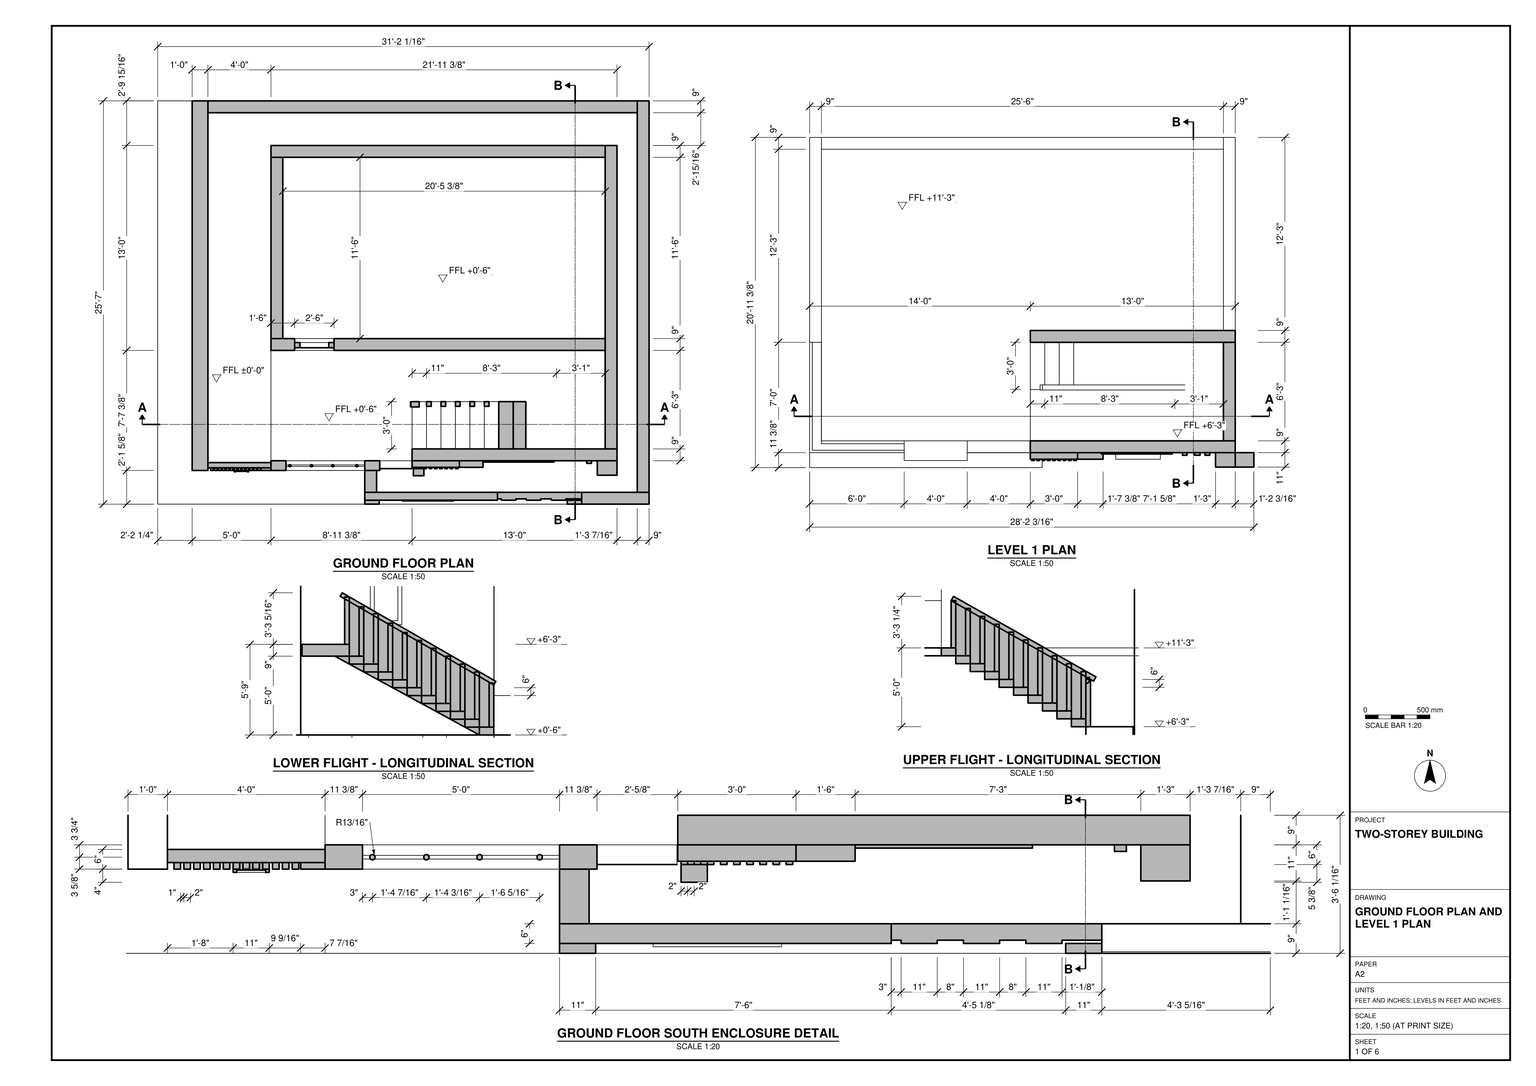
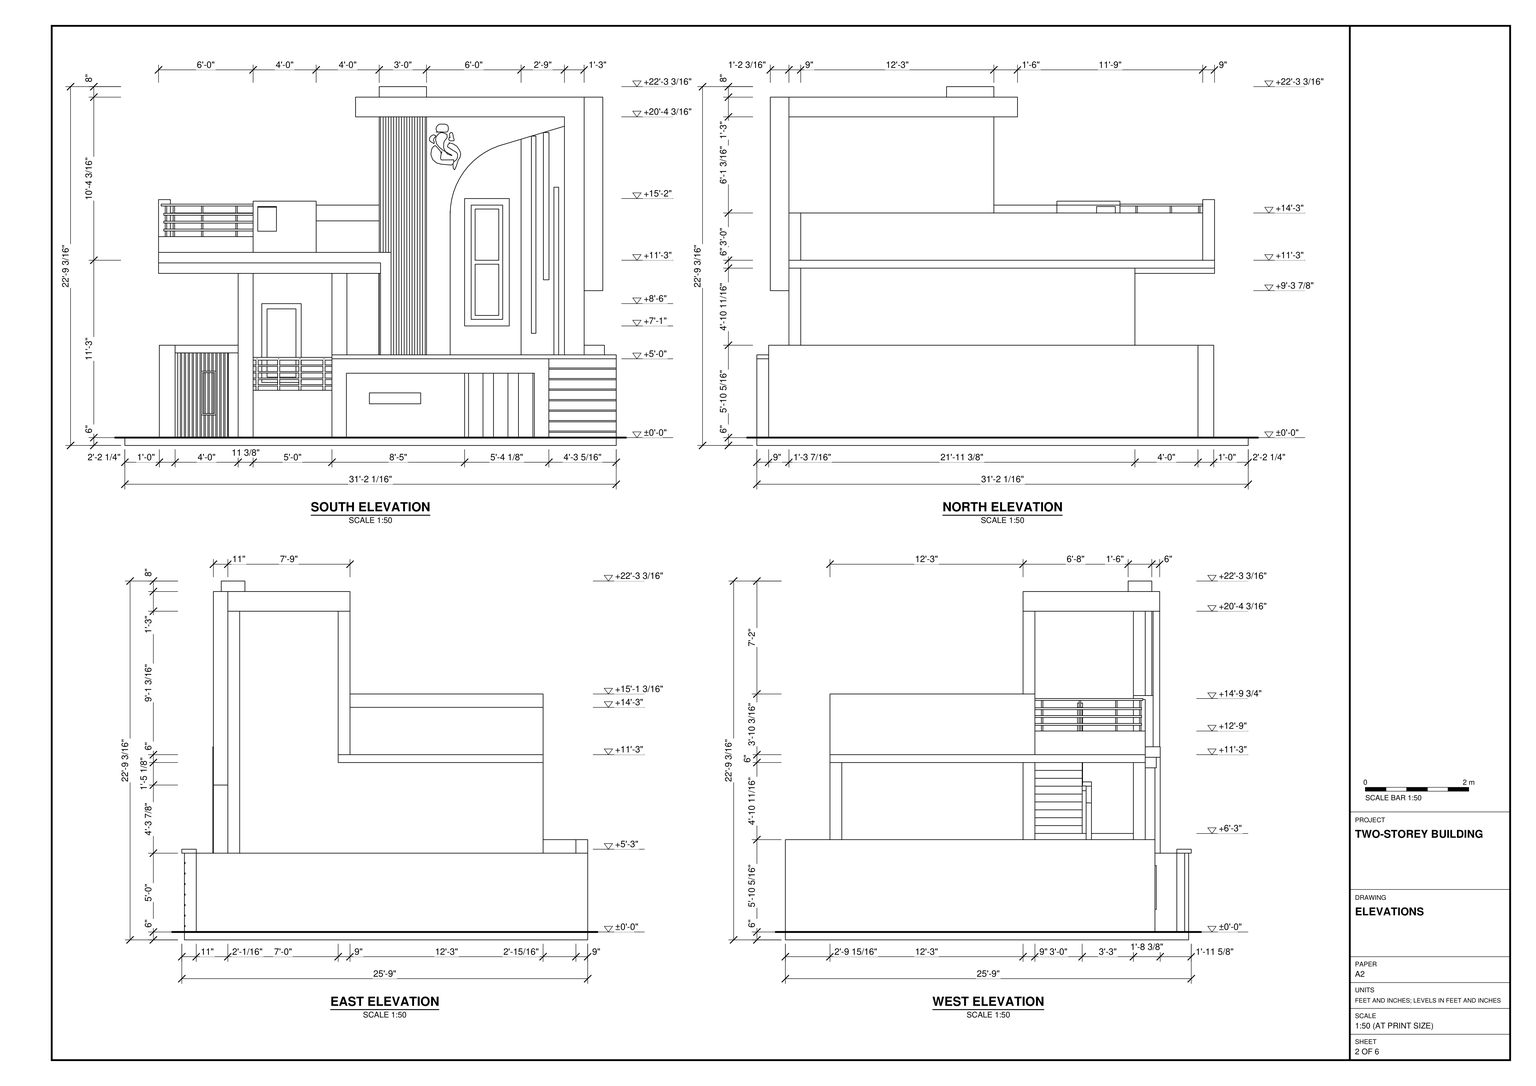
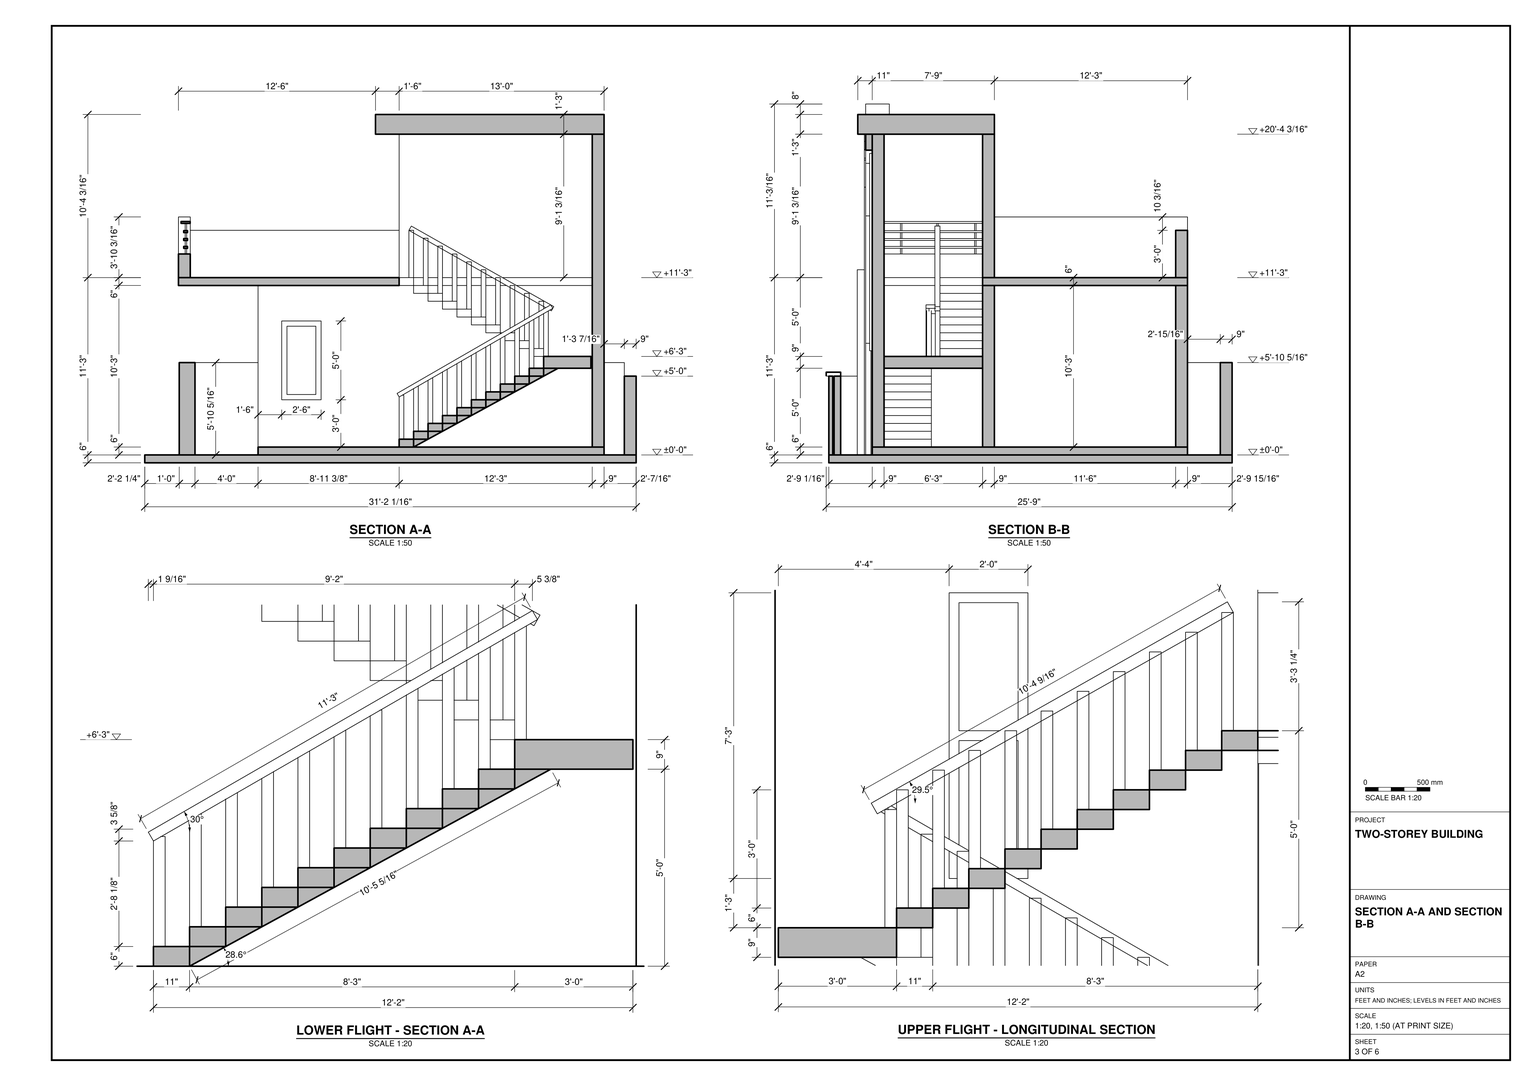
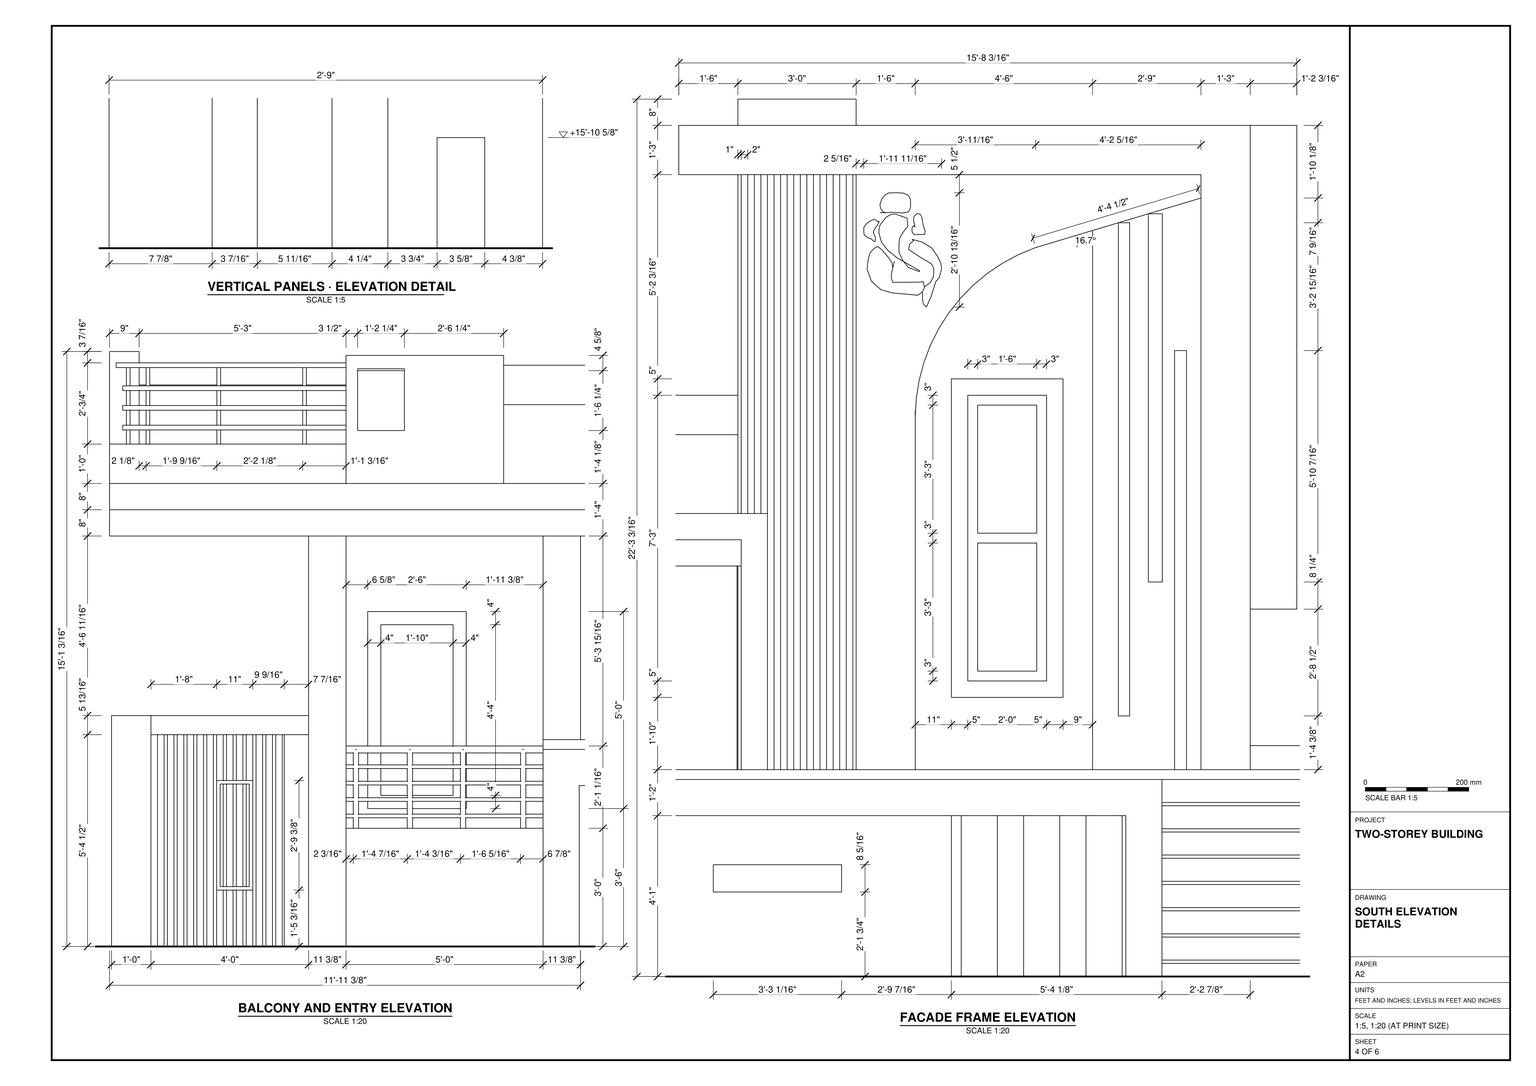
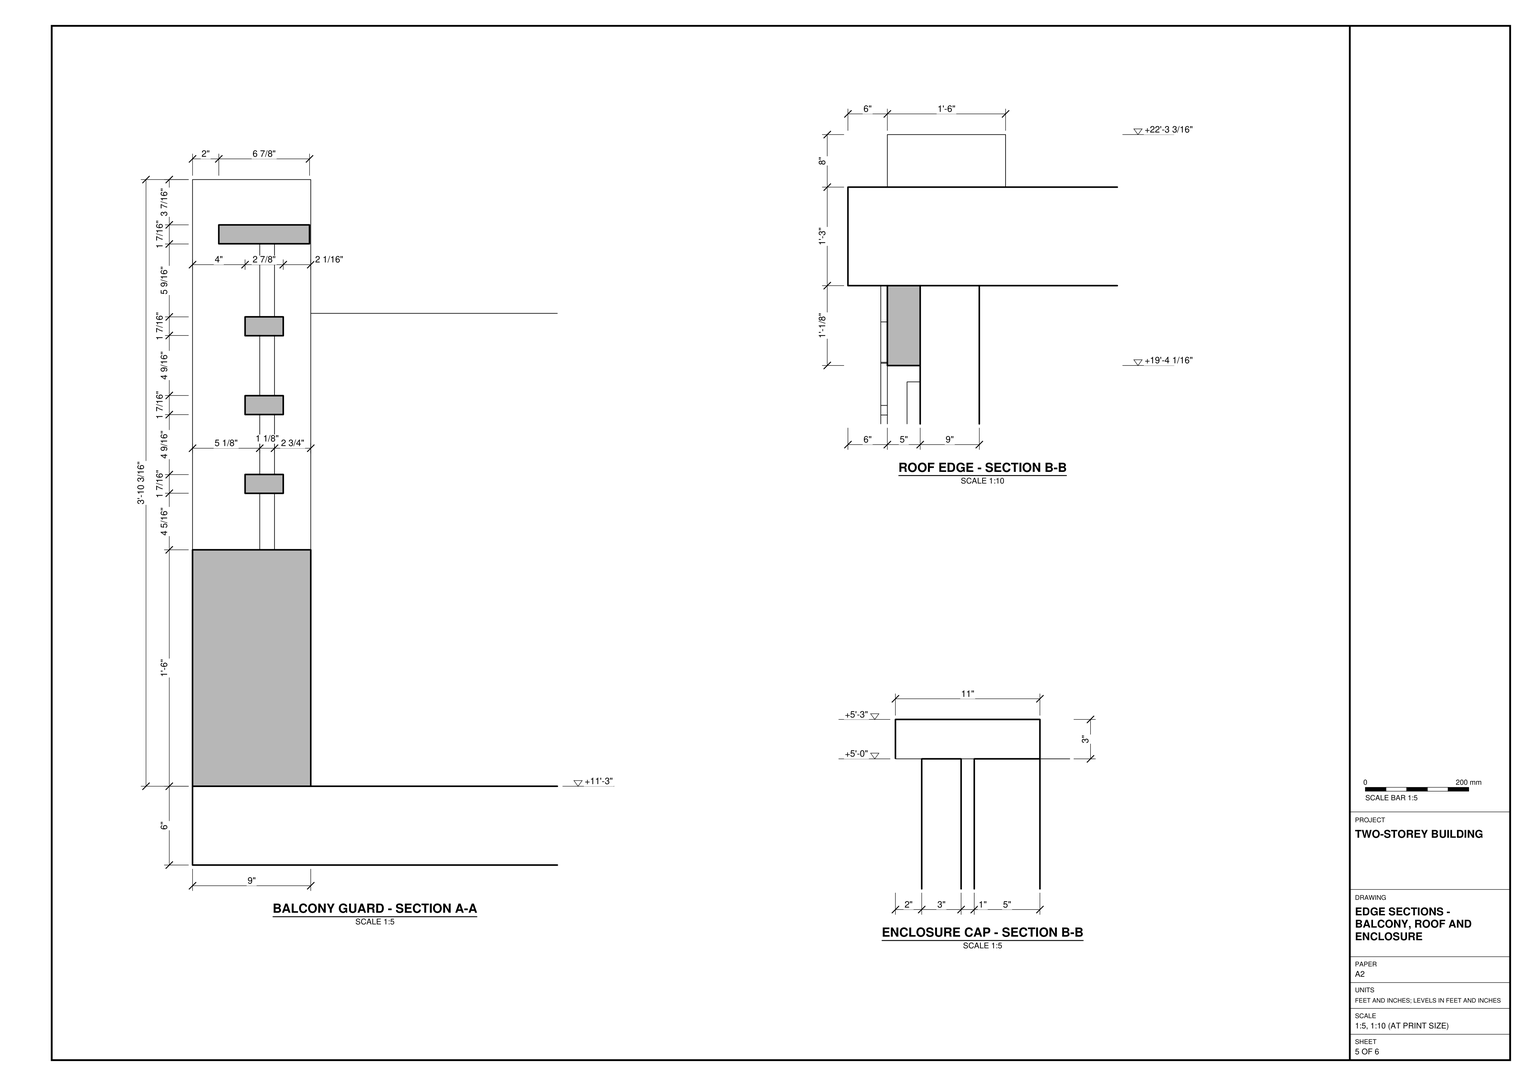
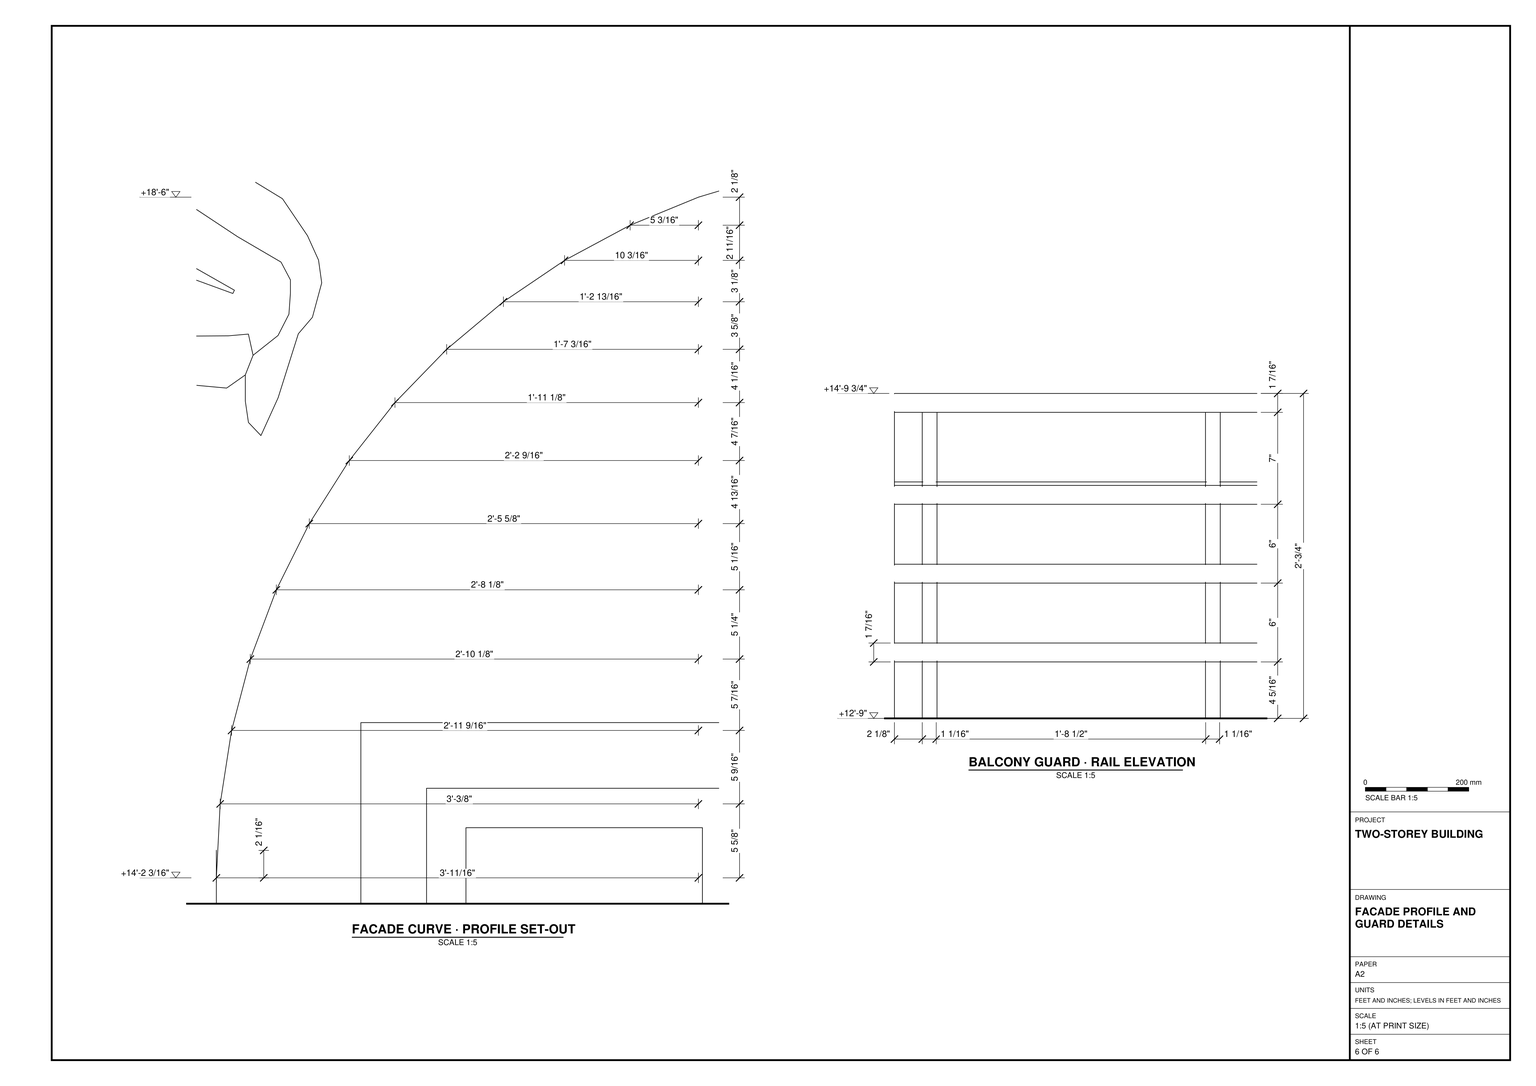
Build the two-storey building in SketchUp from task_files/diagram_01.pdf. Work in feet and inches. Set the overall east–west width to 31'-2 1/16", the north–south depth to 25'-9", and the overall height to 22'-9 3/16". Use ±0'-0" as the ground datum and +11'-3" as the upper floor level.

Use the ground floor plan to lay out the perimeter walls, the raised floor at +0'-6", the rectangular rear enclosure and the stair bay along its south wall. Follow the wall and slab thicknesses shown in plan and section. Place the framed opening in the wall beside the stair. Build the lower flight up to the landing at +6'-3", then reverse direction for the upper flight to the terrace. Include the treads, sloping handrails and vertical balusters.

Keep the terrace open apart from the roof over the stair bay. Match the solid parapets and horizontal railings to the elevations. On the south face, model the tall curved-edge panel, narrow framed window and projecting roof edge behind the low front enclosure. Distinguish the slatted gate and railed bay from the solid panels of that enclosure.

Make the walls, slabs, roof, stair assemblies and any furniture or joinery pieces separate groups or components, and use components for repeated parts. Decor and loose items shown may be represented by any suitable library component. Save one SketchUp model as output_files/two_storey_building_with_a_return_stair_and_terrace.skp.

# SketchUp Ruby script. Lengths in inches.
U = 1.inch
M = Sketchup.active_model
def pt(a) = Geom::Point3d.new(a.map { |v| v * U })
def face(e, loops, mat)
  f = e.add_face(loops[0].map { |a| pt(a) })
  loops[1..].each { |l| e.add_face(l.map { |a| pt(a) }).erase! }
  f.material = f.back_material = mat if mat
  f
end
# faces: each face lists its corners as indices into pts; further lists are holes
def faces(e, pts, list, mat = nil) = list.each { |f| face(e, (f[0].is_a?(Array) ? f : [f]).map { |l| l.map { |i| pts[i] } }, mat) }
# xy, xz, yz: faces in a plane at the given z, y or x. An outline is a flat list of corners, or four numbers for a rectangle; further outlines are holes
def ring(l) = l.size == 4 ? [[l[0], l[1]], [l[2], l[1]], [l[2], l[3]], [l[0], l[3]]] : l.each_slice(2).to_a
def flat(e, list, mat, &to3) = list.each { |f| face(e, (f[0].is_a?(Array) ? f : [f]).map { |l| ring(l).map { |u, v| to3.(u, v) } }, mat) }
def xy(e, z, list, mat = nil) = flat(e, list, mat) { |x, y| [x, y, z] }
def xz(e, y, list, mat = nil) = flat(e, list, mat) { |x, z| [x, y, z] }
def yz(e, x, list, mat = nil) = flat(e, list, mat) { |y, z| [x, y, z] }
def lines(e, pts, list) = list.each { |a, b| e.add_line(pt(pts[a]), pt(pts[b])) }
# prism: a flat outline (further loops are holes) pulled along v
def prism(e, loops, v, mat = nil)
  f = face(e, loops, mat); d = Geom::Vector3d.new(v.map { |x| x * U })
  f.pushpull(f.normal.samedirection?(d) ? d.length : -d.length)
end
def box(e, o, s, mat = nil) = prism(e, [[o, [o[0] + s[0], o[1], o[2]], [o[0] + s[0], o[1] + s[1], o[2]], [o[0], o[1] + s[1], o[2]]]], [0, 0, s[2]], mat)
def at(x, y, z, deg = 0) = Geom::Transformation.translation(pt([x, y, z])) * Geom::Transformation.rotation(ORIGIN, Z_AXIS, deg.degrees)
def axes(o, x, y, z) = Geom::Transformation.new([*x, 0, *y, 0, *z, 0, *pt(o).to_a, 1])
def part(name) = M.definitions.add(name)
# library, detail: a bought-in or finely detailed component or shape, given as its bounding box
def library(name, o, s) = part(name).tap { |d| box(d.entities, o, s) }
def detail(e, o, s) = box(e.add_group.entities, o, s)
def put(e, d, t, mat = nil) = e.add_instance(d, t).tap { |i| i.material = mat if mat }
def group(e, t, mat = nil) = e.add_group.tap { |g| g.transformation = t; g.material = mat if mat }.entities
root = M.entities
M.materials.add("[Aluminum]").color = [179, 179, 179]
M.materials.add("[Color B08]").color = [102, 25, 0]
M.materials.add("[Color C01]").color = [255, 229, 204]
M.materials.add("[Color C02]").color = [255, 204, 153]
M.materials.add("[Color E03]").color = [255, 255, 101]
M.materials.add("[Color M00]").color = [255, 255, 255]
M.materials.add("[Color M05]").color = [114, 114, 114]
M.materials.add("[Color M07]").color = [58, 58, 58]
M.materials.add("[Color M08]").color = [30, 30, 30]
M.materials.add("[Color M09]").color = [0, 0, 0]
M.materials.add("[Translucent Glass Gray]").color = [128, 128, 128]
M.materials["[Translucent Glass Gray]"].alpha = 0.5
M.materials.add("[Wood Veneer 01]").color = [58, 34, 18]
c1 = part("Group\#9")
box(c1.entities,[0,0,0],[11,36,6])
c2 = part("Group\#12")
box(c2.entities,[0,0,0],[11,36,6])
c3 = part("Group\#19")
box(c3.entities,[0,0,0],[3.5625,3.5625,36])
c4 = part("Group\#30")
box(c4.entities,[0,0,0],[2,1,244.1875])
c5 = part("Group\#43")
prism(c5.entities,[[[1.6,1.02,0],[1.625,0.8125,0],[1.6,0.6,0],[1.52,0.41,0],[1.39,0.24,0],[1.22,0.11,0],[1.02,0.03,0],[0.8125,0,0],[0.6,0.03,0],[0.41,0.11,0],[0.24,0.24,0],[0.11,0.41,0],[0.03,0.6,0],[0,0.8125,0],[0.03,1.02,0],[0.11,1.22,0],[0.24,1.39,0],[0.41,1.52,0],[0.6,1.6,0],[0.8125,1.625,0],[1.02,1.6,0],[1.22,1.52,0],[1.39,1.39,0],[1.52,1.22,0]]],[0,0,24])
c6 = part("Group\#45")
prism(c6.entities,[[[62.1875,0,0.5],[62.1875,0.04,0.35],[62.1875,0.11,0.22],[62.1875,0.21,0.12],[62.1875,0.33,0.04],[62.1875,0.48,0],[62.1875,0.62,0],[62.1875,0.76,0.04],[62.1875,0.89,0.11],[62.1875,1,0.21],[62.1875,1.07,0.33],[62.1875,1.12,0.48],[62.1875,1.12,0.62],[62.1875,1.08,0.76],[62.1875,1.01,0.89],[62.1875,0.91,1],[62.1875,0.78,1.07],[62.1875,0.64,1.12],[62.1875,0.5,1.12],[62.1875,0.35,1.08],[62.1875,0.22,1.01],[62.1875,0.12,0.91],[62.1875,0.04,0.78],[62.1875,0,0.64]]],[-62.1875,0,0])
c7 = part("Group\#57")
prism(c7.entities,[[[22,0.25,0.93],[22,0.15,0.85],[22,0.07,0.75],[22,0.02,0.63],[22,0,0.5],[22,0.02,0.37],[22,0.07,0.25],[22,0.15,0.15],[22,0.25,0.07],[22,0.37,0.02],[22,0.5,0],[22,0.63,0.02],[22,0.75,0.07],[22,0.85,0.15],[22,0.93,0.25],[22,0.98,0.37],[22,1,0.5],[22,0.98,0.63],[22,0.93,0.75],[22,0.85,0.85],[22,0.75,0.93],[22,0.63,0.98],[22,0.5,1],[22,0.37,0.98]]],[-22,0,0])
c8 = part("Group\#58")
prism(c8.entities,[[[70,2.9375,0],[70,1,0],[2,1,0],[2,82.16,0],[4.91,82.16,0],[4.91,2.9375,0]]],[0,0,1.4375])
c9 = part("Group\#60")
prism(c9.entities,[[[0.01,0.4375,0],[0,0.58,0],[0.02,0.73,0],[0.09,0.86,0],[0.18,0.98,0],[0.3,1.06,0],[0.4375,1.11,0],[0.58,1.125,0],[0.73,1.1,0],[0.86,1.04,0],[0.98,0.94,0],[1.06,0.82,0],[1.11,0.6875,0],[1.125,0.54,0],[1.1,0.4,0],[1.04,0.26,0],[0.94,0.15,0],[0.82,0.0625,0],[0.6875,0.01,0],[0.54,0,0],[0.4,0.02,0],[0.26,0.09,0],[0.15,0.18,0],[0.0625,0.3,0]]],[0,0,23.3])
c10 = part("Group\#69")
box(c10.entities,[0,0,0],[2,2,64.5])
c11 = library("Group\#76",[0,0,0],[26.62,2,36.65])
xz(root,29.04,[[169.04,42,193.38,135]],"[Translucent Glass Gray]")
g1 = group(root,at(72,2,0))
box(g1,[-72,0,0],[374.0625,307,6])
g2 = group(root,at(109.64,35.04,6))
box(g2,[-23.4,0,0],[263.4,240,6])
g3 = group(root,at(229.64,35.04,12),"[Color C02]")
prism(g3,[[[-36,0,0],[120,0,0],[120,0,238.1875],[-36,0,238.1875]],[[58,0,84],[34,0,84],[34,0,171],[58,0,171]]],[0,9,0])
g4 = group(root,at(340.64,44.04,12),"[Color C01]")
prism(g4,[[[0,231,0],[0,0,0],[0,0,238.1875],[0,75,238.1875],[0,75,123],[0,231,123]]],[9,0,0])
g5 = group(root,at(109.64,266.04,12),"[Color C01]")
box(g5,[-23.4,0,0],[254.4,9,123])
g6 = group(root,at(109.64,119.04,12),"[Color C01]")
prism(g6,[[[231,9,0],[-23.4,9,0],[-23.4,9,123],[231,9,123]],[[-5.4,9,36],[24.6,9,36],[24.6,9,96],[-5.4,9,96]]],[0,-9,0])
g7 = group(root,at(193.64,44.04,12))
xy(g7,6,[[11,0,22,36]])
xy(g7,12,[[22,0,33,36]])
xy(g7,18,[[33,0,44,36]])
xy(g7,24,[[44,0,55,36]])
xy(g7,30,[[55,0,66,36]])
xy(g7,36,[[66,0,77,36]])
xy(g7,42,[[77,0,88,36]])
xy(g7,48,[[88,0,99,36]])
xy(g7,54,[[99,0,110,36]])
xy(g7,60,[[110,0,121,36]])
xz(g7,0,[[11,0,22,6,11,6],[22,6,33,12,22,12],[33,12,44,18,33,18],[44,18,55,24,44,24],[55,24,66,30,55,30],
  [66,30,77,36,66,36],[77,36,88,42,77,42],[88,42,99,48,88,48],[99,48,110,54,99,54],[110,54,121,60,110,60]])
xz(g7,36,[[11,0,11,6,22,6],[22,6,22,12,33,12],[33,12,33,18,44,18],[44,18,44,24,55,24],[55,24,55,30,66,30],
  [66,30,66,36,77,36],[77,36,77,42,88,42],[88,42,88,48,99,48],[99,48,99,54,110,54],[110,54,110,60,121,60]])
yz(g7,11,[[0,0,36,6]])
yz(g7,22,[[0,6,36,12]])
yz(g7,33,[[0,12,36,18]])
yz(g7,44,[[0,18,36,24]])
yz(g7,55,[[0,24,36,30]])
yz(g7,66,[[0,30,36,36]])
yz(g7,77,[[0,36,36,42]])
yz(g7,88,[[0,42,36,48]])
yz(g7,99,[[0,48,36,54]])
yz(g7,110,[[0,54,36,60]])
p = [[11,36,0],[22,36,6],[22,0,6],[11,0,0],[33,36,12],[33,0,12],
  [44,36,18],[44,0,18],[55,36,24],[55,0,24],[66,36,30],[66,0,30],
  [77,36,36],[77,0,36],[88,36,42],[88,0,42],[99,36,48],[99,0,48],
  [110,36,54],[110,0,54],[121,36,60],[121,0,60]]
faces(g7,p,[[0,1,2,3],[1,4,5,2],[4,6,7,5],[6,8,9,7],[8,10,11,9],[10,12,13,11],[12,14,15,13],[14,16,17,15],
  [16,18,19,17],[18,20,21,19]])
put(g7,c1,at(22,0,12))
put(g7,c1,at(11,0,6))
put(g7,c1,at(44,0,24))
put(g7,c1,at(88,0,48))
put(g7,c1,at(0,0,0))
put(g7,c1,at(77,0,42))
put(g7,c1,at(99,0,54))
put(g7,c1,at(55,0,30))
put(g7,c1,at(66,0,36))
put(g7,c1,at(33,0,18))
g8 = group(root,at(303.64,44.04,72))
box(g8,[0,0,0],[36,75,9])
g9 = group(root,at(193.64,83.04,81))
put(g9,c2,at(99,0,0))
put(g9,c2,at(44,0,30))
put(g9,c2,at(55,0,24))
put(g9,c2,at(88,0,6))
put(g9,c2,at(77,0,12))
put(g9,c2,at(11,0,48))
put(g9,c2,at(66,0,18))
put(g9,c2,at(33,0,36))
put(g9,c2,at(22,0,42))
put(g9,c2,at(0,0,54))
g10 = group(root,at(109.64,119.04,135),"[Color C01]")
prism(g10,[[[240,0,0],[84,0,0],[84,-84,0],[-84,-84,0],[-84,156,0],[240,156,0]]],[0,0,6])
g11 = group(root,at(193.64,76.47,18),"[Color M07]")
box(g11,[0,0,0],[3.5625,3.5625,33.5])
put(root,c3,at(204.64,76.47,24),"[Color M07]")
put(root,c3,at(215.64,76.47,30),"[Color M07]")
put(root,c3,at(226.64,76.47,36),"[Color M07]")
put(root,c3,at(237.64,76.47,42),"[Color M07]")
put(root,c3,at(248.64,76.47,48),"[Color M07]")
put(root,c3,at(259.64,76.47,54),"[Color M07]")
g12 = group(root,at(270.64,76.47,60),"[Color M07]")
box(g12,[0,0,0],[3.5625,3.5625,37.0625])
g13 = group(root,at(281.64,76.47,66),"[Color M07]")
box(g13,[0,0,0],[3.5625,3.5625,38.28])
g14 = group(root,at(292.64,76.47,72),"[Color M07]")
box(g14,[0,0,0],[3.5625,3.5625,37.5])
put(root,c3,at(303.64,76.47,81),"[Color M07]")
put(root,c3,at(303.64,83.04,81),"[Color M07]")
put(root,c3,at(300.08,83.04,87),"[Color M07]")
put(root,c3,at(289.08,83.04,93),"[Color M07]")
put(root,c3,at(278.08,83.04,99),"[Color M07]")
put(root,c3,at(267.08,83.04,105),"[Color M07]")
put(root,c3,at(256.08,83.04,111),"[Color M07]")
put(root,c3,at(245.08,83.04,117),"[Color M07]")
put(root,c3,at(234.08,83.04,123),"[Color M07]")
put(root,c3,at(223.08,83.04,129),"[Color M07]")
put(root,c3,at(212.08,83.04,135),"[Color M07]")
put(root,c3,at(201.08,83.04,141),"[Color M07]")
g15 = group(root,at(192.08,76.47,50.125),"[Color M07]")
xz(g15,-0.5,[[1.5625,0,0,2.71,116.95,70.16,118.51,67.45]])
xz(g15,3.5625,[[1.5625,0,111.5625,63.45,111.5625,67.06,0,2.71]])
xz(g15,6.5625,[[114.16,64.94,118.51,67.45,116.95,70.16,114.16,68.55]])
xz(g15,6.75,[[111.5625,63.45,114.16,64.94,114.16,68.55,111.5625,67.06]])
yz(g15,111.5625,[[3.5625,63.45,6.75,67.06]])
yz(g15,114.16,[[6.5625,64.94,6.75,68.55]])
p = [[0,-0.5,2.71],[1.5625,-0.5,0],[1.5625,1.78,0],[1.5625,3.5625,0],[0,3.5625,2.71],[118.51,-0.5,67.45],
  [118.51,1.78,67.45],[118.51,6.5625,67.45],[114.16,6.5625,64.94],[114.16,6.75,64.94],[111.5625,6.75,63.45],[111.5625,3.5625,63.45],
  [111.5625,3.5625,67.06],[111.5625,6.75,67.06],[114.16,6.75,68.55],[114.16,6.5625,68.55],[116.95,6.5625,70.16],[116.95,-0.5,70.16]]
faces(g15,p,[[0,1,2,3,4],[1,5,6,2],[3,2,6,7,8,9,10,11],[0,4,12,13,14,15,16,17],[5,17,16,7,6]])
g16 = group(root,at(201.08,83.04,117),"[Color M07]")
prism(g16,[[[108.44,3.5625,-1.31],[110.28,3.5625,1.94],[110.28,-0.3,1.94],[108.44,-0.3,-1.31],[108.44,1.78,-1.31]]],[-108.44,0,61.31])
g17 = group(root,at(193.64,119.04,141),"[Color C01]")
box(g17,[0,0,0],[156,9,109.1875])
g18 = group(root,at(340.64,128.04,141),"[Color C01]")
box(g18,[0,0,0],[9,147,36])
g19 = group(root,at(109.64,266.04,141),"[Color C01]")
box(g19,[-75,0,0],[306,9,36])
g20 = group(root,at(331.64,29.04,6),"[Color B08]")
xy(g20,0,[[3,-5,18,6]])
xy(g20,244.1875,[[-156,-5,-156,99,0,99,0,6,3,6,3,-5],[0,6,18,99]])
xy(g20,259.1875,[[-156,-5,18,99]])
xz(g20,-5,[[3,0,18,0,18,259.1875,-156,259.1875,-156,244.1875,3,244.1875]])
xz(g20,6,[[3,0,18,244.1875]])
xz(g20,99,[[-156,244.1875,18,259.1875]])
yz(g20,-156,[[-5,244.1875,99,259.1875]])
yz(g20,3,[[-5,0,6,244.1875]])
yz(g20,18,[[-5,0,6,0,6,244.1875,99,244.1875,99,259.1875,-5,259.1875]])
g21 = group(root,at(247.64,30.04,6),"[Color C01]")
g22 = group(g21,at(0,4,0))
prism(g22,[[[54,0,0],[54,0,244.1875],[0,0,244.1875],[0,0,0]],[[40,0,90],[16,0,90],[16,0,177],[40,0,177]]],[0,1,0])
g23 = group(g21,at(11,0,85))
prism(g23,[[[34,5,0],[0,5,0],[0,5,97],[34,5,97]],[[5,5,92],[5,5,5],[29,5,5],[29,5,92]]],[0,-5,0],"[Color M00]")
g24 = group(root,at(193.64,30.04,6),"[Color C02]")
xy(g24,0,[[0,0,36,5],[36,0,54,5]])
xy(g24,244.1875,[[0,0,36,5],[36,0,141,5]])
xz(g24,0,[[0,0,36,244.1875],[36,0,54,0,54,170.1875,54.29,175.82,55.15,181.39,56.59,186.84,58.57,192.12,61.08,197.17,64.1,201.93,67.59,206.36,71.52,210.41,75.84,214.03,80.51,217.19,85.48,219.86,90.69,222,141,237.07,141,244.1875,36,244.1875]])
xz(g24,5,[[0,0,36,244.1875],[36,0,36,244.1875,141,244.1875,141,237.07,90.69,222,85.48,219.86,80.51,217.19,75.84,214.03,71.52,210.41,67.59,206.36,64.1,201.93,61.08,197.17,58.57,192.12,56.59,186.84,55.15,181.39,54.29,175.82,54,170.1875,54,0]])
yz(g24,0,[[0,0,5,244.1875]])
yz(g24,36,[[0,0,5,244.1875]])
yz(g24,54,[[0,0,5,170.1875]])
yz(g24,141,[[0,237.07,5,244.1875]])
p = [[54,5,170.1875],[54.29,5,175.82],[54.29,0,175.82],[54,0,170.1875],[55.15,5,181.39],[55.15,0,181.39],
  [56.59,5,186.84],[56.59,0,186.84],[58.57,5,192.12],[58.57,0,192.12],[61.08,5,197.17],[61.08,0,197.17],
  [64.1,5,201.93],[64.1,0,201.93],[67.59,5,206.36],[67.59,0,206.36],[71.52,5,210.41],[71.52,0,210.41],
  [75.84,5,214.03],[75.84,0,214.03],[80.51,5,217.19],[80.51,0,217.19],[85.48,5,219.86],[85.48,0,219.86],
  [90.69,5,222],[90.69,0,222],[141,5,237.07],[141,0,237.07],[141,5,0],[54,5,0]]
faces(g24,p,[[0,1,2,3],[1,4,5,2],[4,6,7,5],[6,8,9,7],[8,10,11,9],[10,12,13,11],[12,14,15,13],[14,16,17,15],
  [16,18,19,17],[18,20,21,19],[20,22,23,21],[22,24,25,23],[24,26,27,25]])
lines(g24,p,[[26,28],[28,29]])
put(root,c4,at(194.64,29.04,6),"[Color C01]")
put(root,c4,at(198.64,29.04,6),"[Color C01]")
put(root,c4,at(202.64,29.04,6),"[Color C01]")
put(root,c4,at(206.64,29.04,6),"[Color C01]")
put(root,c4,at(210.64,29.04,6),"[Color C01]")
put(root,c4,at(214.64,29.04,6),"[Color C01]")
put(root,c4,at(218.64,29.04,6),"[Color C01]")
put(root,c4,at(222.64,29.04,6),"[Color C01]")
put(root,c4,at(226.64,29.04,6),"[Color C01]")
g25 = group(root,at(263.64,34.04,96),"[Color M09]")
prism(g25,[[[0,3,0],[0,3,87],[24,3,87],[24,3,0]],[[21,3,42],[3,3,42],[3,3,3],[21,3,3]],[[3,3,84],[3,3,45],[21,3,45],[21,3,84]]],[0,-3,0])
g26 = group(root,at(266.64,34.04,99),"[Translucent Glass Gray]")
xz(g26,0,[[0,0,18,39]])
g27 = group(root,at(266.64,34.04,141),"[Translucent Glass Gray]")
xz(g27,0,[[0,0,18,39]])
g28 = group(root,at(193.64,30.04,265.1875),"[Color C01]")
box(g28,[0,0,0],[36,18,8])
g29 = group(root,at(109.64,35.04,141),"[Color M00]")
box(g29,[-12,0,0],[96,9,42],"[Color E03]")
g30 = group(root,at(86.24,23.64,6),"[Color C01]")
prism(g30,[[[11.4,11.4,0],[0,11.4,0],[0,11.4,129],[11.4,11.4,129],[11.4,11.4,36]]],[0,-7.4,0])
g31 = group(root,at(157.64,23.64,6),"[Color C01]")
prism(g31,[[[11.4,11.4,0],[0,11.4,0],[0,11.4,129],[11.4,11.4,129],[11.4,11.4,36]]],[0,-7.4,0])
g32 = group(root,at(97.64,23.64,6),"[Color C01]")
box(g32,[0,4,0],[60,7.4,36])
g33 = group(root,at(25.64,23.64,135),"[Color C01]")
box(g33,[0,3,-4],[169,8.4,8])
g34 = group(root,at(169.04,29.04,6))
box(g34,[0,0,0],[24.34,6,36])
g35 = group(root,at(25.64,23.64,6),"[Color B08]")
xy(g35,0,[[169,0,177,5.4]])
xy(g35,133,[[0,0,169,11.4],[169,5.4,177,11.4]])
xy(g35,141,[[0,0,177,11.4]])
xz(g35,0,[[169,0,177,0,177,141,0,141,0,133,169,133]])
xz(g35,5.4,[[169,0,177,133]])
xz(g35,11.4,[[0,133,169,141],[169,133,177,141]])
yz(g35,0,[[0,133,11.4,141]])
yz(g35,169,[[0,0,5.4,133]])
yz(g35,177,[[0,0,5.4,0,5.4,133,11.4,133,11.4,141,0,141]])
put(root,c5,at(99.84,30.46,42),"[Color M07]")
g36 = group(root,at(116.28,30.46,42),"[Color M07]")
prism(g36,[[[1.6,1.02,0],[1.625,0.8125,0],[1.6,0.6,0],[1.52,0.41,0],[1.39,0.24,0],[1.22,0.11,0],[1.02,0.03,0],[0.8125,0,0],[0.6,0.03,0],[0.41,0.11,0],[0.24,0.24,0],[0.11,0.41,0],[0.03,0.6,0],[0,0.8125,0],[0.03,1.02,0],[0.11,1.22,0],[0.24,1.39,0],[0.41,1.52,0],[0.6,1.6,0],[0.8125,1.625,0],[1.02,1.6,0],[1.22,1.52,0],[1.39,1.39,0],[1.52,1.22,0]]],[0,0,24])
put(root,c5,at(132.46,30.46,42),"[Color M07]")
put(root,c5,at(150.78,30.46,42),"[Color M07]")
g37 = group(root,at(97.64,30.21,64.9375),"[Color M07]")
prism(g37,[[[0,1.0625,2.125],[0,1.34,2.09],[0,1.59,1.98],[0,1.8125,1.8125],[0,1.98,1.59],[0,2.09,1.34],[0,2.125,1.0625],[0,2.09,0.79],[0,1.98,0.53],[0,1.8125,0.3125],[0,1.59,0.14],[0,1.34,0.04],[0,1.0625,0],[0,0.79,0.04],[0,0.53,0.14],[0,0.3125,0.3125],[0,0.14,0.53],[0,0.04,0.79],[0,0,1.0625],[0,0.04,1.34],[0,0.14,1.59],[0,0.3125,1.8125],[0,0.53,1.98],[0,0.79,2.09]]],[60,0,0])
put(root,c6,at(97.64,30.71,60.19),"[Color M07]")
put(root,c6,at(97.64,30.71,55.19),"[Color M07]")
put(root,c6,at(97.64,30.71,50.19),"[Color M07]")
put(root,c6,at(97.64,30.71,45.19),"[Color M07]")
put(root,c6,at(97.64,30.71,40.19))
g38 = group(root,at(157.64,2,6),"[Color E03]")
box(g38,[0,3,0],[101,6,60])
g39 = group(root,at(157.64,2,6),"[Color B08]")
prism(g39,[[[165.125,3,60],[165.125,3,0],[154.125,3,0],[154.125,3,49],[11,3,49],[11,3,0],[0,3,0],[0,3,60]]],[0,-3,0])
g40 = group(root,at(258.64,5,6),"[Color C01]")
xy(g40,0,[[3,0,3,1,0,1,0,6,64.125,6,64.125,1,52,1,52,0,41,0,41,1,33,1,33,0,22,0,22,1,14,1,14,0]])
xy(g40,60,[[3,0,14,0,14,1,22,1,22,0,33,0,33,1,41,1,41,0,52,0,52,1,64.125,1,64.125,6,0,6,0,1,3,1]])
xz(g40,0,[[3,0,14,60],[22,0,33,60],[41,0,52,60]],"[Color C02]")
xz(g40,1,[[0,0,3,60],[14,0,22,60],[33,0,41,60],[52,0,64.125,60]])
xz(g40,6,[[0,0,64.125,60]])
yz(g40,0,[[1,0,6,60]])
yz(g40,3,[[0,0,1,60]])
yz(g40,14,[[0,0,1,60]])
yz(g40,22,[[0,0,1,60]])
yz(g40,33,[[0,0,1,60]])
yz(g40,41,[[0,0,1,60]])
yz(g40,52,[[0,0,1,60]])
yz(g40,64.125,[[1,0,6,60]])
g41 = group(root,at(322.76,2,6),"[Color C02]")
prism(g41,[[[51.3,9,0],[51.3,9,60],[51.3,0,60],[51.3,0,53],[51.3,0.5,53],[51.3,0.5,52],[51.3,0,52],[51.3,0,45],[51.3,0.5,45],[51.3,0.5,44],[51.3,0,44],[51.3,0,37],[51.3,0.5,37],[51.3,0.5,36],[51.3,0,36],[51.3,0,29],[51.3,0.5,29],[51.3,0.5,28],[51.3,0,28],[51.3,0,21],[51.3,0.5,21],[51.3,0.5,20],[51.3,0,20],[51.3,0,13],[51.3,0.5,13],[51.3,0.5,12],[51.3,0,12],[51.3,0,5],[51.3,0.5,5],[51.3,0.5,4],[51.3,0,4],[51.3,0,0]]],[-51.3,0,0])
g42 = group(root,at(157.64,0,6),"[Color C01]")
xy(g42,0,[[0,11,9,27.64]])
xy(g42,60,[[0,11,9,27.64]])
xy(g42,63,[[0,0,216.42,11]])
xz(g42,0,[[0,60,216.42,63]])
xz(g42,11,[[0,0,9,60],[0,60,9,63],[9,60,216.42,63]])
xz(g42,27.64,[[0,0,9,60]])
yz(g42,0,[[11,0,27.64,60],[0,60,11,63]])
yz(g42,9,[[11,0,27.64,60]])
yz(g42,216.42,[[0,60,11,63]])
g43 = group(root,at(365.0625,11,6),"[Color C01]")
box(g43,[0,0,0],[9,298,60])
g44 = group(root,at(72,300,6),"[Color C01]")
box(g44,[-33.76,0,0],[326.82,9,70.3125])
g45 = group(root,at(97.64,29.04,147),"[Color C02]")
prism(g45,[[[48,15,39],[48,15,0],[0,15,0],[0,15,39]],[[3.52,15,16.11],[17.77,15,16.11],[17.77,15,34.93],[3.52,15,34.93]]],[0,-15,0])
g46 = group(root,at(145.64,34.9375,171),"[Color C01]")
box(g46,[0,0,0],[48,0.1,12])
g47 = group(root,at(101.16,34.9375,163.11),"[Color E03]")
box(g47,[0,0,0],[14.25,0.1,18.25])
g48 = group(root,at(25.64,35.04,141),"[Color C01]")
prism(g48,[[[72,9,0],[72,0,0],[0,0,0],[0,84,0],[9,84,0],[9,9,0]]],[0,0,18])
g49 = group(root,at(25.64,119.04,141),"[Color C01]")
box(g49,[0,0,0],[9,156,46.1875])
g50 = group(root,at(104.24,121.04,48),"[Wood Veneer 01]")
prism(g50,[[[0,0,60],[0,0,0],[30,0,0],[30,0,60]],[[26,0,56],[26,0,4],[4,0,4],[4,0,56]]],[0,4,0])
put(root,c7,at(108.24,122.54,100.5),"[Aluminum]")
put(root,c7,at(108.24,122.54,97.5),"[Aluminum]")
put(root,c7,at(108.24,122.54,94.5),"[Aluminum]")
put(root,c7,at(108.24,122.54,91.5),"[Aluminum]")
put(root,c7,at(108.24,122.54,88.5),"[Aluminum]")
put(root,c7,at(108.24,122.54,85.5),"[Aluminum]")
put(root,c7,at(108.24,122.54,82.5),"[Aluminum]")
put(root,c7,at(108.24,122.54,79.5),"[Aluminum]")
put(root,c7,at(108.24,122.54,76.5),"[Aluminum]")
put(root,c7,at(108.24,122.54,73.5),"[Aluminum]")
put(root,c7,at(108.24,122.54,70.5),"[Aluminum]")
put(root,c7,at(108.24,122.54,67.5),"[Aluminum]")
put(root,c7,at(108.24,122.54,64.5),"[Aluminum]")
put(root,c7,at(108.24,122.54,61.5),"[Aluminum]")
put(root,c7,at(108.24,122.54,58.5),"[Aluminum]")
put(root,c7,at(108.24,122.54,55.5),"[Aluminum]")
put(root,c7,at(108.24,122.54,49.5))
put(root,c7,at(108.24,122.54,46.5))
g51 = group(root,at(27.64,36.88,182.3),"[Color M07]")
prism(g51,[[[70,4.9375,0],[70,0,0],[0,0,0],[0,82.16,0],[6.91,82.16,0],[6.91,4.9375,0]]],[0,0,1.4375])
put(root,c8,at(27.64,36.88,175.3),"[Color M07]")
put(root,c8,at(27.64,36.88,169.3),"[Color M07]")
put(root,c8,at(27.64,36.88,163.3),"[Color M07]")
put(root,c9,at(30.75,56.5,159),"[Color M07]")
put(root,c9,at(36.75,38.25,159),"[Color M07]")
put(root,c9,at(58.32,38.25,159),"[Color M07]")
put(root,c9,at(84.44,38.25,159),"[Color M07]")
put(root,c9,at(30.75,84.19,159),"[Color M07]")
put(root,c9,at(30.75,112.94,159),"[Color M07]")
g52 = group(root,at(38.24,29.64,6))
xy(g52,0,[[0,0,48,4]],"[Color M09]")
xy(g52,64.5,[[0,0,48,4]],"[Color M09]")
xz(g52,0,[[0,0,48,64.5]],"[Color M05]")
xz(g52,4,[[0,0,48,64.5]],"[Color M09]")
yz(g52,0,[[0,0,4,64.5]],"[Color M09]")
yz(g52,48,[[0,0,4,64.5]],"[Color M09]")
put(root,c10,at(40.24,27.64,6),"[Color M08]")
put(root,c10,at(43.24,27.64,6),"[Color M08]")
put(root,c10,at(46.24,27.64,6),"[Color M08]")
put(root,c10,at(49.24,27.64,6),"[Color M08]")
g53 = group(root,at(52.24,27.64,6),"[Color M08]")
box(g53,[0,0,0],[2,2,64.5])
put(root,c10,at(55.24,27.64,6),"[Color M08]")
put(root,c10,at(58.24,27.64,6),"[Color M08]")
g54 = group(root,at(61.24,27.64,6),"[Color M08]")
box(g54,[0,0,0],[2,2,64.5])
g55 = group(root,at(64.24,27.64,6),"[Color M08]")
box(g55,[0,0,0],[2,2,64.5])
put(root,c10,at(67.24,27.64,6),"[Color M08]")
put(root,c10,at(70.24,27.64,6),"[Color M08]")
put(root,c10,at(73.24,27.64,6),"[Color M08]")
put(root,c10,at(76.24,27.64,6),"[Color M08]")
g56 = group(root,at(78.8125,27.64,6),"[Color M08]")
box(g56,[0,0,0],[7.42,2,64.5])
g57 = group(root,at(58.24,26.64,23.16),"[Color M07]")
xy(g57,0,[[0,0,11,1]])
xy(g57,1.08,[[1.08,0,9.92,0.7],[1.08,0.7,9.92,1]])
xy(g57,32.3125,[[1.08,0,9.92,0.7],[1.08,0.7,9.92,1]])
xy(g57,33.39,[[0,0,11,1]])
xz(g57,0,[[[0,0,11,33.39],[1.08,1.08,9.92,32.3125]]])
xz(g57,0.7,[[1.08,1.08,9.92,32.3125]],"[Color M05]")
xz(g57,1,[[[0,0,11,33.39],[1.08,1.08,9.92,32.3125]]])
yz(g57,0,[[0,0,1,33.39]])
yz(g57,1.08,[[0,1.08,0.7,32.3125],[0.7,1.08,1,32.3125]])
yz(g57,9.92,[[0,1.08,0.7,32.3125],[0.7,1.08,1,32.3125]])
yz(g57,11,[[0,0,1,33.39]])
g58 = group(root,at(26.24,27.64,6),"[Color C01]")
box(g58,[0,0,0],[12,281.36,70.3125])
g59 = group(root,at(86.24,128.04,12),"[Color C01]")
box(g59,[0,0,0],[9,138,123])
g60 = group(root,at(349.64,24.04,117.875),"[Color C01]")
box(g60,[0,0,0],[14.1875,11,147.3125])
g61 = group(root,at(186.14,4,31.73))
box(g61,[0,0,0],[39.0625,1,8.3125])
g62 = group(root,at(108.24,121.04,52),"[Translucent Glass Gray]")
xz(g62,0,[[0,0,22,52]])
g63 = group(root,at(309.49,33.04,85.35))
box(g63,[0,0,0],[3.4375,2,150.1875])
g64 = group(root,at(318.61,33.04,126.14))
box(g64,[0,0,0],[4.25,2,112.125])
g65 = group(root,at(327.67,33.04,21.36))
box(g65,[-1.0625,0,0],[3.625,2,175.25])
put(root,c11,axes([231.97,29.04,209.85],[0.89,0,0],[0,1,0],[0,0,0.95]))
